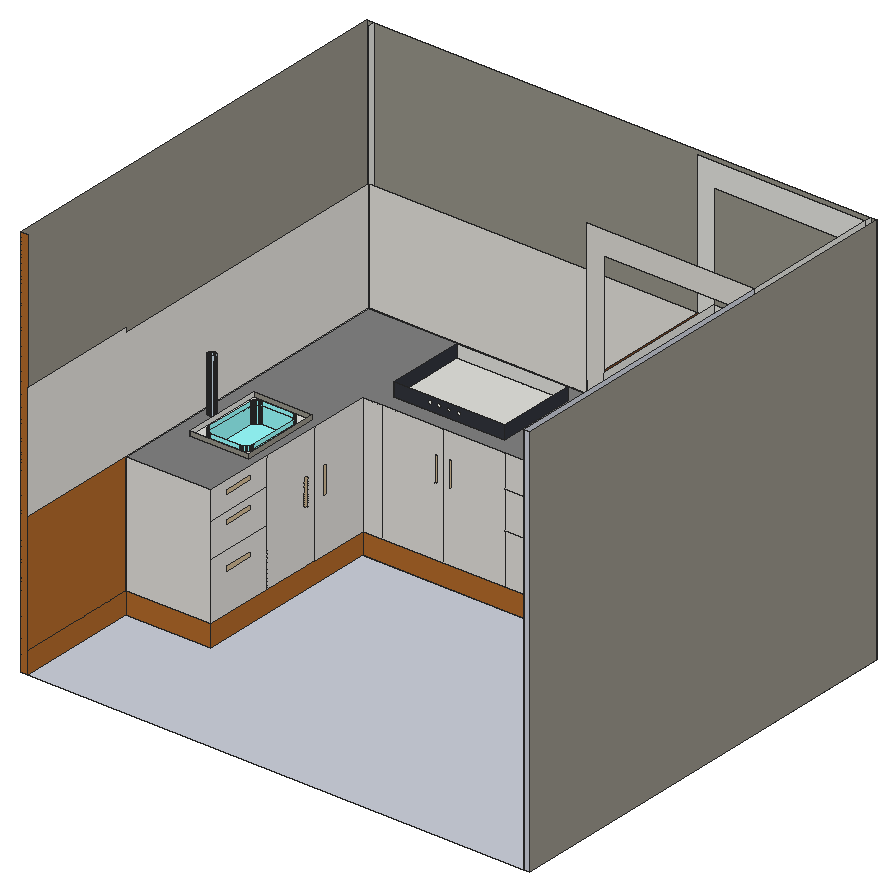
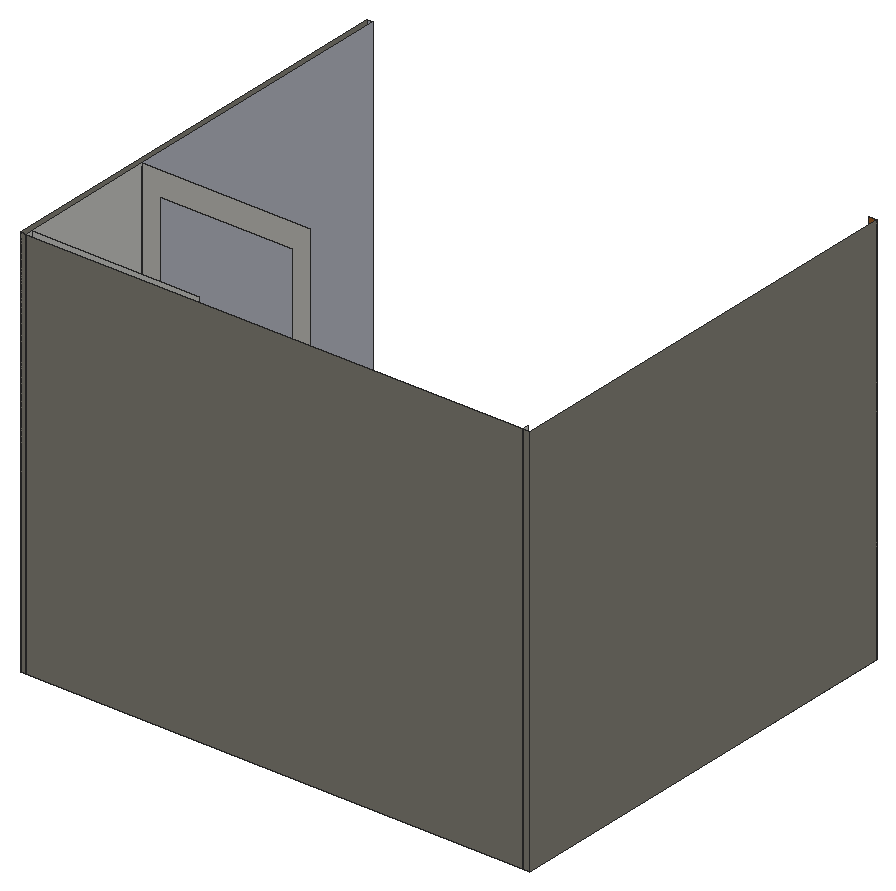
# SketchUp Ruby script. Lengths in inches.
U = 1.inch
M = Sketchup.active_model
def pt(a) = Geom::Point3d.new(a.map { |v| v * U })
def face(e, loops, mat)
  f = e.add_face(loops[0].map { |a| pt(a) })
  loops[1..].each { |l| e.add_face(l.map { |a| pt(a) }).erase! }
  f.material = f.back_material = mat if mat
  f
end
# faces: each face lists its corners as indices into pts; further lists are holes
def faces(e, pts, list, mat = nil) = list.each { |f| face(e, (f[0].is_a?(Array) ? f : [f]).map { |l| l.map { |i| pts[i] } }, mat) }
# xy, xz, yz: faces in a plane at the given z, y or x. An outline is a flat list of corners, or four numbers for a rectangle; further outlines are holes
def ring(l) = l.size == 4 ? [[l[0], l[1]], [l[2], l[1]], [l[2], l[3]], [l[0], l[3]]] : l.each_slice(2).to_a
def flat(e, list, mat, &to3) = list.each { |f| face(e, (f[0].is_a?(Array) ? f : [f]).map { |l| ring(l).map { |u, v| to3.(u, v) } }, mat) }
def xy(e, z, list, mat = nil) = flat(e, list, mat) { |x, y| [x, y, z] }
def xz(e, y, list, mat = nil) = flat(e, list, mat) { |x, z| [x, y, z] }
def yz(e, x, list, mat = nil) = flat(e, list, mat) { |y, z| [x, y, z] }
def lines(e, pts, list) = list.each { |a, b| e.add_line(pt(pts[a]), pt(pts[b])) }
# prism: a flat outline (further loops are holes) pulled along v
def prism(e, loops, v, mat = nil)
  f = face(e, loops, mat); d = Geom::Vector3d.new(v.map { |x| x * U })
  f.pushpull(f.normal.samedirection?(d) ? d.length : -d.length)
end
def box(e, o, s, mat = nil) = prism(e, [[o, [o[0] + s[0], o[1], o[2]], [o[0] + s[0], o[1] + s[1], o[2]], [o[0], o[1] + s[1], o[2]]]], [0, 0, s[2]], mat)
def at(x, y, z, deg = 0) = Geom::Transformation.translation(pt([x, y, z])) * Geom::Transformation.rotation(ORIGIN, Z_AXIS, deg.degrees)
def axes(o, x, y, z) = Geom::Transformation.new([*x, 0, *y, 0, *z, 0, *pt(o).to_a, 1])
def part(name) = M.definitions.add(name)
# library, detail: a bought-in or finely detailed component or shape, given as its bounding box
def library(name, o, s) = part(name).tap { |d| box(d.entities, o, s) }
def detail(e, o, s) = box(e.add_group.entities, o, s)
def put(e, d, t, mat = nil) = e.add_instance(d, t).tap { |i| i.material = mat if mat }
def group(e, t, mat = nil) = e.add_group.tap { |g| g.transformation = t; g.material = mat if mat }.entities
root = M.entities
M.materials.add("[Color H02]").color = [153, 255, 255]
M.materials.add("[Formica Beige]").color = [211, 187, 149]
M.materials.add("[Formica Graystone]").color = [149, 146, 135]
M.materials.add("[Formica Laminate Dark]").color = [50, 53, 60]
M.materials.add("[Herringbone]").color = [130, 130, 130]
M.materials.add("[Marble Carrara Floor Tile]").color = [204, 208, 219]
M.materials.add("[Marble Carrara Gold Floor Tile]").color = [225, 223, 217]
M.materials.add("[Terrazzo Light Blue]").color = [196, 214, 227]
M.materials.add("[Terrazzo Tile Accent]").color = [224, 221, 217]
M.materials.add("[Terrazzo Tile Light]").color = [219, 217, 210]
M.materials.add("[Wood Bamboo]").color = [177, 105, 43]
M.materials.add("[Wood Veneer 01]").color = [120, 70, 37]
xy(root,0,[[0,0,0,133.25,2.25,133.25,2.25,96,28.4375,96,28.4375,37.75,2.25,37.75,2.25,0],[154.9375,0,156.6875,133.25],[103.5,87.9375,103.5,96,2.25,96,2.25,131.0625,154.9375,131.0625,154.9375,87.9375],[2.25,131.0625,154.9375,133.25]])
xy(root,0,[[2.25,0,2.25,37.75,28.4375,37.75,28.4375,96,103.5,96,103.5,87.9375,154.9375,87.9375,154.9375,0]],"[Marble Carrara Floor Tile]")
xy(root,6.5625,[[2.25,37.75,28.4375,96],[103.5,87.9375,108.5,88.5625],[108.5,87.9375,149.5,88.5625],[149.5,87.9375,154.9375,88.5625],[103.5,88.5625,108.5,131.0625],
  [108.5,88.5625,149.5,131.0625],[149.5,88.5625,154.9375,131.0625],[2.25,96,23.375,131.0625],[23.375,96,103.5,131.0625]])
xy(root,38.4375,[[12.63,57.43,21.47,57.43,21.78,57.45,22.09,57.51,22.39,57.61,22.68,57.75,22.94,57.93,23.18,58.14,23.39,58.375,23.57,58.64,23.71,58.93,23.81,59.23,23.87,59.54,23.89,59.85,23.89,75.31,23.87,75.61,23.8125,75.9,23.72,76.1875,23.58,76.46,23.42,76.71,23.22,76.9375,22.99,77.14,22.74,77.3,22.47,77.4375,22.18,77.53,21.89,77.59,21.58,77.61,12.11,77.61,11.83,77.6,11.57,77.54,11.31,77.45,11.0625,77.33,10.84,77.18,10.63,77,10.45,76.8,10.3,76.57,10.18,76.33,10.09,76.07,10.04,75.8,10.02,75.53,10.02,60.04,10.04,59.7,10.11,59.36,10.22,59.04,10.37,58.73,10.56,58.45,10.78,58.19,11.04,57.97,11.33,57.78,11.63,57.625,11.96,57.52,12.29,57.45]],"[Color H02]")
xy(root,42.13,[[108.5,88.5625,149.5,92.5]],"[Formica Laminate Dark]")
xy(root,43.5,[[[7.92,55.33,25.99,79.71],[12.63,57.43,21.47,57.43,21.78,57.45,22.09,57.51,22.39,57.61,22.68,57.75,22.94,57.93,23.18,58.14,23.39,58.375,23.57,58.64,23.71,58.93,23.81,59.23,23.87,59.54,23.89,59.85,23.89,75.31,23.87,75.61,23.8125,75.9,23.72,76.1875,23.58,76.46,23.42,76.71,23.22,76.9375,22.99,77.14,22.74,77.3,22.47,77.4375,22.18,77.53,21.89,77.59,21.58,77.61,12.11,77.61,11.83,77.6,11.57,77.54,11.31,77.45,11.0625,77.33,10.84,77.18,10.63,77,10.45,76.8,10.3,76.57,10.18,76.33,10.09,76.07,10.04,75.8,10.02,75.53,10.02,60.04,10.04,59.7,10.11,59.36,10.22,59.04,10.37,58.73,10.56,58.45,10.78,58.19,11.04,57.97,11.33,57.78,11.63,57.625,11.96,57.52,12.29,57.45]],[5.01,66.11,4.71,66.15,4.42,66.27,4.17,66.45,3.99,66.7,3.87,66.99,3.83,67.29,3.87,67.6,3.99,67.89,4.17,68.13,4.42,68.32,4.71,68.44,5.01,68.48,5.32,68.44,5.61,68.32,5.85,68.13,6.04,67.89,6.16,67.6,6.2,67.29,6.16,66.99,6.04,66.7,5.85,66.45,5.61,66.27,5.32,66.15],[34.11,101.1,68.05,125.35]])
xy(root,43.5,[[[2.25,37.75,28.4375,37.75,28.4375,96,103.5,96,103.5,131.0625,2.25,131.0625],[34.11,101.1,68.05,125.35],[7.92,55.33,25.99,79.71],[5.01,66.11,4.71,66.15,4.42,66.27,4.17,66.45,3.99,66.7,3.87,66.99,3.83,67.29,3.87,67.6,3.99,67.89,4.17,68.13,4.42,68.32,4.71,68.44,5.01,68.48,5.32,68.44,5.61,68.32,5.85,68.13,6.04,67.89,6.16,67.6,6.2,67.29,6.16,66.99,6.04,66.7,5.85,66.45,5.61,66.27,5.32,66.15]]],"[Herringbone]")
xz(root,0,[[154.9375,0,156.6875,121.1875]],"[Marble Carrara Floor Tile]")
xz(root,0,[[0,0,2.25,121.1875]],"[Wood Bamboo]")
xz(root,37.75,[[2.25,6.5625,28.4375,43.5]],"[Terrazzo Tile Accent]")
xz(root,37.75,[[2.25,0,28.4375,6.5625]],"[Wood Bamboo]")
xz(root,55.33,[[7.92,43.5,25.99,44.875]],"[Formica Graystone]")
xz(root,57.43,[[12.63,38.4375,21.47,43.5],[12.63,43.5,21.47,44.875]],"[Color H02]")
xz(root,77.61,[[12.11,38.4375,21.58,43.5],[12.11,43.5,21.58,44.875]],"[Color H02]")
xz(root,79.71,[[7.92,43.5,25.99,44.875]],"[Formica Graystone]")
xz(root,87.9375,[[103.5,0,154.9375,6.5625]],"[Formica Graystone]")
xz(root,88.5625,[[108.5,6.5625,149.5,42.13]],"[Formica Graystone]")
xz(root,88.5625,[[103.5,6.5625,108.5,6.5625,108.5,113.88,149.5,113.88,149.5,6.5625,154.9375,6.5625,154.9375,121.1875,103.5,121.1875]],"[Terrazzo Tile Light]")
xz(root,92.5,[[108.5,42.13,149.5,46.64]],"[Formica Laminate Dark]")
xz(root,96,[[2.25,0,28.4375,6.5625]])
xz(root,96,[[81.29,16.72,96.81,18.52],[50.66,27.79,51.73,35.85],[54.91,27.79,55.98,35.85],[81.29,29.34,96.81,31.14],[81.29,39.22,96.81,41.02]],"[Formica Beige]")
xz(root,96,[[28.4375,6.5625,34.39,43.5],[[34.39,6.5625,53.25,43.5],[50.66,27.79,51.73,35.85]],[[53.25,6.5625,72.1,43.5],[54.91,27.79,55.98,35.85]],[[72.1,6.5625,103.5,22.18],[81.29,16.72,96.81,18.52]],[[72.1,22.18,103.5,33.77],[81.29,29.34,96.81,31.14]],
  [[72.1,33.77,103.5,43.5],[81.29,39.22,96.81,41.02]]],"[Terrazzo Tile Accent]")
xz(root,96,[[28.4375,0,103.5,6.5625]],"[Wood Bamboo]")
xz(root,101.1,[[[34.11,43.5,68.05,47.5],[45.19,45.12,45.02,45.14,44.85,45.21,44.71,45.32,44.6,45.46,44.53,45.625,44.51,45.8,44.53,45.98,44.6,46.15,44.71,46.29,44.85,46.4,45.02,46.47,45.19,46.49,45.37,46.47,45.54,46.4,45.68,46.29,45.79,46.15,45.86,45.98,45.88,45.8,45.86,45.625,45.79,45.46,45.68,45.32,45.54,45.21,45.37,45.14],[54.07,45.12,53.89,45.14,53.72,45.21,53.58,45.32,53.47,45.46,53.4,45.625,53.38,45.8,53.4,45.98,53.47,46.15,53.58,46.29,53.72,46.4,53.89,46.47,54.07,46.49,54.25,46.47,54.41,46.4,54.55,46.29,54.66,46.15,54.73,45.98,54.76,45.8,54.73,45.625,54.66,45.46,54.55,45.32,54.41,45.21,54.25,45.14],[48.01,45.12,47.83,45.14,47.66,45.21,47.52,45.32,47.41,45.46,47.34,45.625,47.32,45.8,47.34,45.98,47.41,46.15,47.52,46.29,47.66,46.4,47.83,46.47,48.01,46.49,48.18,46.47,48.35,46.4,48.49,46.29,48.6,46.15,48.67,45.98,48.69,45.8,48.67,45.625,48.6,45.46,48.49,45.32,48.35,45.21,48.18,45.14],[50.88,45.12,50.7,45.14,50.54,45.21,50.39,45.32,50.29,45.46,50.22,45.625,50.19,45.8,50.22,45.98,50.29,46.15,50.39,46.29,50.54,46.4,50.7,46.47,50.88,46.49,51.06,46.47,51.22,46.4,51.37,46.29,51.48,46.15,51.55,45.98,51.57,45.8,51.55,45.625,51.48,45.46,51.37,45.32,51.22,45.21,51.06,45.14]]],"[Formica Laminate Dark]")
xz(root,125.35,[[34.11,43.5,68.05,47.5]])
xz(root,131.0625,[[2.25,0,154.9375,6.5625],[2.25,6.5625,23.375,43.5],[23.375,6.5625,103.5,43.5],[103.5,6.5625,103.5,121.1875,154.9375,121.1875,154.9375,6.5625,149.5,6.5625,149.5,113.88,108.5,113.88,108.5,6.5625],[108.5,6.5625,149.5,81.6875]])
xz(root,131.0625,[[2.25,43.5,103.5,77.75]],"[Marble Carrara Gold Floor Tile]")
xz(root,133.25,[[0,0,2.25,121.1875],[2.25,0,154.9375,121.1875],[154.9375,0,156.6875,121.1875]],"[Formica Graystone]")
yz(root,0,[[0,0,133.25,121.1875]],"[Formica Graystone]")
yz(root,2.25,[[96,0,131.0625,6.5625],[131.0625,0,133.25,121.1875],[37.75,6.5625,131.0625,43.5]])
yz(root,2.25,[[0,43.5,131.0625,43.5,131.0625,77.75,37.75,77.75,37.75,79.12,0,79.12]],"[Marble Carrara Gold Floor Tile]")
yz(root,2.25,[[0,0,37.75,6.5625],[0,6.5625,37.75,43.5]],"[Wood Bamboo]")
yz(root,7.92,[[55.33,43.5,79.71,44.875]])
yz(root,10.02,[[60.04,38.4375,75.53,43.5],[60.04,43.5,75.53,44.875]],"[Color H02]")
yz(root,23.89,[[59.85,38.4375,75.31,43.5],[59.85,43.5,75.31,44.875]],"[Color H02]")
yz(root,25.99,[[55.33,43.5,79.71,44.875]],"[Formica Graystone]")
yz(root,28.4375,[[43.4,18.31,53.15,20.06],[73.36,22.6875,74.93,31.5625],[80.8,22.6875,82.36,31.5625],[43.4,31.25,53.15,33],[43.4,39.5,53.15,41.25]],"[Formica Beige]")
yz(root,28.4375,[[[37.75,6.5625,59.25,24.35],[43.4,18.31,53.15,20.06]],[[59.25,6.5625,77.625,43.5],[73.36,22.6875,74.93,31.5625]],[[77.625,6.5625,96,43.5],[80.8,22.6875,82.36,31.5625]],[[37.75,24.35,59.25,34.89],[43.4,31.25,53.15,33]],[[37.75,34.89,59.25,43.5],[43.4,39.5,53.15,41.25]]],"[Terrazzo Tile Accent]")
yz(root,28.4375,[[37.75,0,96,6.5625]],"[Wood Bamboo]")
yz(root,34.11,[[101.1,43.5,125.35,47.5]],"[Formica Laminate Dark]")
yz(root,68.05,[[101.1,43.5,125.35,47.5]],"[Formica Laminate Dark]")
yz(root,103.5,[[87.9375,0,96,6.5625],[96,6.5625,131.0625,43.5]])
yz(root,103.5,[[88.5625,6.5625,96,43.5],[88.5625,43.5,131.0625,77.75]],"[Wood Veneer 01]")
yz(root,108.5,[[88.5625,6.5625,131.0625,6.5625,131.0625,81.6875,88.5625,81.6875,88.5625,46.64,92.5,46.64,92.5,42.13,88.5625,42.13]])
yz(root,108.5,[[88.5625,42.13,92.5,46.64]],"[Formica Laminate Dark]")
yz(root,149.5,[[88.5625,6.5625,88.5625,42.13,92.5,42.13,92.5,46.64,88.5625,46.64,88.5625,81.6875,131.0625,81.6875,131.0625,6.5625]])
yz(root,149.5,[[88.5625,42.13,92.5,46.64]],"[Formica Laminate Dark]")
yz(root,154.9375,[[87.9375,0,131.0625,6.5625],[131.0625,0,133.25,121.1875],[88.5625,6.5625,131.0625,121.1875]])
yz(root,154.9375,[[0,0,0,121.1875,88.5625,121.1875,88.5625,6.5625,87.9375,6.5625,87.9375,0]],"[Marble Carrara Floor Tile]")
yz(root,156.6875,[[0,0,133.25,121.1875]],"[Formica Graystone]")
p = [[11.96,57.52,43.5],[12.29,57.45,43.5],[12.29,57.45,38.4375],[11.96,57.52,38.4375],[12.63,57.43,43.5],[12.63,57.43,38.4375],
  [21.47,57.43,43.5],[21.78,57.45,43.5],[21.78,57.45,38.4375],[21.47,57.43,38.4375],[22.09,57.51,43.5],[22.09,57.51,38.4375],
  [11.63,57.625,43.5],[11.63,57.625,38.4375],[22.39,57.61,43.5],[22.39,57.61,38.4375],[11.33,57.78,43.5],[11.33,57.78,38.4375],
  [22.68,57.75,43.5],[22.68,57.75,38.4375],[11.04,57.97,43.5],[11.04,57.97,38.4375],[22.94,57.93,43.5],[22.94,57.93,38.4375],
  [23.18,58.14,43.5],[23.18,58.14,38.4375],[10.78,58.19,43.5],[10.78,58.19,38.4375],[23.39,58.375,43.5],[23.39,58.375,38.4375],
  [10.56,58.45,43.5],[10.56,58.45,38.4375],[10.37,58.73,43.5],[10.37,58.73,38.4375],[23.57,58.64,43.5],[23.57,58.64,38.4375],
  [23.71,58.93,43.5],[23.71,58.93,38.4375],[10.22,59.04,43.5],[10.22,59.04,38.4375],[23.81,59.23,43.5],[23.81,59.23,38.4375],
  [10.11,59.36,43.5],[10.11,59.36,38.4375],[23.87,59.54,43.5],[23.87,59.54,38.4375],[10.04,59.7,43.5],[10.04,59.7,38.4375],
  [23.89,59.85,43.5],[23.89,59.85,38.4375],[10.02,60.04,43.5],[10.02,60.04,38.4375],[23.89,75.31,43.5],[23.87,75.61,43.5],
  [23.87,75.61,38.4375],[23.89,75.31,38.4375],[10.04,75.8,43.5],[10.02,75.53,43.5],[10.02,75.53,38.4375],[10.04,75.8,38.4375],
  [23.8125,75.9,43.5],[23.8125,75.9,38.4375],[10.09,76.07,43.5],[10.09,76.07,38.4375],[23.72,76.1875,43.5],[23.72,76.1875,38.4375],
  [10.18,76.33,43.5],[10.18,76.33,38.4375],[23.58,76.46,43.5],[23.58,76.46,38.4375],[10.3,76.57,43.5],[10.3,76.57,38.4375],
  [23.42,76.71,43.5],[23.42,76.71,38.4375],[10.45,76.8,43.5],[10.45,76.8,38.4375],[23.22,76.9375,43.5],[23.22,76.9375,38.4375],
  [10.63,77,43.5],[10.63,77,38.4375],[22.99,77.14,43.5],[22.99,77.14,38.4375],[10.84,77.18,43.5],[10.84,77.18,38.4375],
  [22.74,77.3,43.5],[22.74,77.3,38.4375],[11.0625,77.33,43.5],[11.0625,77.33,38.4375],[11.31,77.45,43.5],[11.31,77.45,38.4375],
  [22.47,77.4375,43.5],[22.47,77.4375,38.4375],[22.18,77.53,43.5],[22.18,77.53,38.4375],[11.57,77.54,43.5],[11.57,77.54,38.4375],
  [11.83,77.6,43.5],[11.83,77.6,38.4375],[21.89,77.59,43.5],[21.89,77.59,38.4375],[12.11,77.61,43.5],[12.11,77.61,38.4375],
  [21.58,77.61,43.5],[21.58,77.61,38.4375],[11.96,57.52,44.875],[12.29,57.45,44.875],[12.63,57.43,44.875],[21.47,57.43,44.875],
  [21.78,57.45,44.875],[22.09,57.51,44.875],[11.63,57.625,44.875],[22.39,57.61,44.875],[11.33,57.78,44.875],[22.68,57.75,44.875],
  [11.04,57.97,44.875],[22.94,57.93,44.875],[23.18,58.14,44.875],[10.78,58.19,44.875],[23.39,58.375,44.875],[10.56,58.45,44.875],
  [10.37,58.73,44.875],[23.57,58.64,44.875],[23.71,58.93,44.875],[10.22,59.04,44.875],[23.81,59.23,44.875],[10.11,59.36,44.875],
  [23.87,59.54,44.875],[10.04,59.7,44.875],[23.89,59.85,44.875],[10.02,60.04,44.875],[4.42,66.27,43.5],[4.71,66.15,43.5],
  [4.71,66.15,59.875],[4.42,66.27,59.875],[5.01,66.11,43.5],[5.01,66.11,59.875],[5.32,66.15,43.5],[5.32,66.15,59.875],
  [5.61,66.27,43.5],[5.61,66.27,59.875],[4.17,66.45,43.5],[4.17,66.45,59.875],[5.85,66.45,43.5],[5.85,66.45,59.875],
  [3.99,66.7,43.5],[3.99,66.7,59.875],[6.04,66.7,43.5],[6.04,66.7,58.5625],[6.04,66.7,59.875],[3.87,66.99,43.5],
  [3.87,66.99,59.875],[6.16,66.99,43.5],[6.16,66.99,58.5625],[3.83,67.29,43.5],[3.83,67.29,59.875],[6.2,67.29,43.5],
  [6.2,67.29,58.5625],[3.87,67.6,43.5],[3.87,67.6,59.875],[6.16,67.6,43.5],[6.16,67.6,58.5625],[3.99,67.89,43.5],
  [3.99,67.89,59.875],[6.04,67.89,43.5],[6.04,67.89,59.875],[6.16,67.6,59.875],[4.17,68.13,43.5],[4.17,68.13,59.875],
  [5.85,68.13,43.5],[5.85,68.13,59.875],[4.42,68.32,43.5],[4.42,68.32,59.875],[5.61,68.32,43.5],[5.61,68.32,59.875],
  [4.71,68.44,43.5],[4.71,68.44,59.875],[5.32,68.44,43.5],[5.32,68.44,59.875],[5.01,68.48,43.5],[5.01,68.48,59.875],
  [23.89,75.31,44.875],[23.87,75.61,44.875],[10.04,75.8,44.875],[10.02,75.53,44.875],[23.8125,75.9,44.875],[10.09,76.07,44.875],
  [23.72,76.1875,44.875],[10.18,76.33,44.875],[23.58,76.46,44.875],[10.3,76.57,44.875],[23.42,76.71,44.875],[10.45,76.8,44.875],
  [23.22,76.9375,44.875],[10.63,77,44.875],[22.99,77.14,44.875],[10.84,77.18,44.875],[22.74,77.3,44.875],[11.0625,77.33,44.875],
  [11.31,77.45,44.875],[22.47,77.4375,44.875],[22.18,77.53,44.875],[11.57,77.54,44.875],[11.83,77.6,44.875],[21.89,77.59,44.875],
  [12.11,77.61,44.875],[21.58,77.61,44.875]]
faces(root,p,[[0,1,2,3],[1,4,5,2],[6,7,8,9],[7,10,11,8],[12,0,3,13],[10,14,15,11],[16,12,13,17],[14,18,19,15],
  [20,16,17,21],[18,22,23,19],[22,24,25,23],[26,20,21,27],[24,28,29,25],[30,26,27,31],[32,30,31,33],[28,34,35,29],
  [34,36,37,35],[38,32,33,39],[36,40,41,37],[42,38,39,43],[40,44,45,41],[46,42,43,47],[44,48,49,45],[50,46,47,51],
  [52,53,54,55],[56,57,58,59],[53,60,61,54],[62,56,59,63],[60,64,65,61],[66,62,63,67],[64,68,69,65],[70,66,67,71],
  [68,72,73,69],[74,70,71,75],[72,76,77,73],[78,74,75,79],[76,80,81,77],[82,78,79,83],[80,84,85,81],[86,82,83,87],
  [88,86,87,89],[84,90,91,85],[90,92,93,91],[94,88,89,95],[96,94,95,97],[92,98,99,93],[100,96,97,101],[98,102,103,99],
  [1,0,104,105],[4,1,105,106],[7,6,107,108],[10,7,108,109],[0,12,110,104],[14,10,109,111],[12,16,112,110],[18,14,111,113],
  [16,20,114,112],[22,18,113,115],[24,22,115,116],[20,26,117,114],[28,24,116,118],[26,30,119,117],[30,32,120,119],[34,28,118,121],
  [36,34,121,122],[32,38,123,120],[40,36,122,124],[38,42,125,123],[44,40,124,126],[42,46,127,125],[48,44,126,128],[46,50,129,127],
  [53,52,180,181],[57,56,182,183],[60,53,181,184],[56,62,185,182],[64,60,184,186],[62,66,187,185],[68,64,186,188],[66,70,189,187],
  [72,68,188,190],[70,74,191,189],[76,72,190,192],[74,78,193,191],[80,76,192,194],[78,82,195,193],[84,80,194,196],[82,86,197,195],
  [86,88,198,197],[90,84,196,199],[92,90,199,200],[88,94,201,198],[94,96,202,201],[98,92,200,203],[96,100,204,202],[102,98,203,205]],"[Color H02]")
faces(root,p,[[130,131,132,133],[131,134,135,132],[134,136,137,135],[136,138,139,137],[140,130,133,141],[138,142,143,139],[144,140,141,145],[142,146,147,148,143],
  [149,144,145,150],[146,151,152,147],[153,149,150,154],[151,155,156,152],[157,153,154,158],[155,159,160,156],[161,157,158,162],[159,163,164,165,160],
  [166,161,162,167],[163,168,169,164],[170,166,167,171],[168,172,173,169],[174,170,171,175],[172,176,177,173],[178,174,175,179],[176,178,179,177]],"[Terrazzo Light Blue]")
